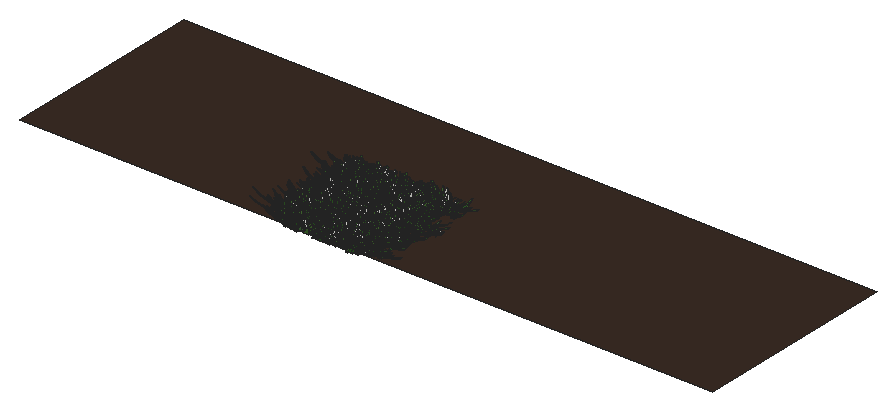
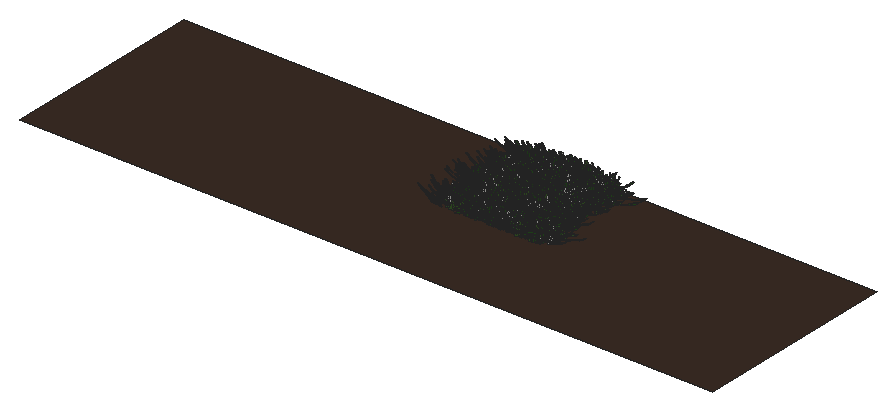
# SketchUp Ruby script. Lengths in inches.
U = 1.inch
M = Sketchup.active_model
def pt(a) = Geom::Point3d.new(a.map { |v| v * U })
def face(e, loops, mat)
  f = e.add_face(loops[0].map { |a| pt(a) })
  loops[1..].each { |l| e.add_face(l.map { |a| pt(a) }).erase! }
  f.material = f.back_material = mat if mat
  f
end
# faces: each face lists its corners as indices into pts; further lists are holes
def faces(e, pts, list, mat = nil) = list.each { |f| face(e, (f[0].is_a?(Array) ? f : [f]).map { |l| l.map { |i| pts[i] } }, mat) }
# xy, xz, yz: faces in a plane at the given z, y or x. An outline is a flat list of corners, or four numbers for a rectangle; further outlines are holes
def ring(l) = l.size == 4 ? [[l[0], l[1]], [l[2], l[1]], [l[2], l[3]], [l[0], l[3]]] : l.each_slice(2).to_a
def flat(e, list, mat, &to3) = list.each { |f| face(e, (f[0].is_a?(Array) ? f : [f]).map { |l| ring(l).map { |u, v| to3.(u, v) } }, mat) }
def xy(e, z, list, mat = nil) = flat(e, list, mat) { |x, y| [x, y, z] }
def xz(e, y, list, mat = nil) = flat(e, list, mat) { |x, z| [x, y, z] }
def yz(e, x, list, mat = nil) = flat(e, list, mat) { |y, z| [x, y, z] }
def lines(e, pts, list) = list.each { |a, b| e.add_line(pt(pts[a]), pt(pts[b])) }
# prism: a flat outline (further loops are holes) pulled along v
def prism(e, loops, v, mat = nil)
  f = face(e, loops, mat); d = Geom::Vector3d.new(v.map { |x| x * U })
  f.pushpull(f.normal.samedirection?(d) ? d.length : -d.length)
end
def box(e, o, s, mat = nil) = prism(e, [[o, [o[0] + s[0], o[1], o[2]], [o[0] + s[0], o[1] + s[1], o[2]], [o[0], o[1] + s[1], o[2]]]], [0, 0, s[2]], mat)
def at(x, y, z, deg = 0) = Geom::Transformation.translation(pt([x, y, z])) * Geom::Transformation.rotation(ORIGIN, Z_AXIS, deg.degrees)
def axes(o, x, y, z) = Geom::Transformation.new([*x, 0, *y, 0, *z, 0, *pt(o).to_a, 1])
def part(name) = M.definitions.add(name)
# library, detail: a bought-in or finely detailed component or shape, given as its bounding box
def library(name, o, s) = part(name).tap { |d| box(d.entities, o, s) }
def detail(e, o, s) = box(e.add_group.entities, o, s)
def put(e, d, t, mat = nil) = e.add_instance(d, t).tap { |i| i.material = mat if mat }
def group(e, t, mat = nil) = e.add_group.tap { |g| g.transformation = t; g.material = mat if mat }.entities
root = M.entities
M.materials.add("Material10").color = [48, 100, 38]
M.materials.add("Material3").color = [68, 110, 58]
M.materials.add("Material4").color = [48, 90, 38]
M.materials.add("Material5").color = [68, 110, 48]
M.materials.add("Material6").color = [48, 90, 48]
M.materials.add("Material7").color = [58, 110, 58]
M.materials.add("Material8").color = [58, 90, 38]
M.materials.add("Material9").color = [68, 100, 58]
M.materials.add("top-soil").color = [58, 44, 36]
c1 = part("grass00")
p = [[-0.6875,0.15,0],[-0.56,0.08,5.52],[-0.04,0.03,2.76],[0.48,-0.02,0],[0.35,-0.02,5.52],[-0.1,-0.14,5.52],
  [-0.12,0.65,8.37],[-0.42,0.65,8.37]]
faces(c1.entities,p,[[0,1,2,3],[3,2,4],[1,5,2],[5,4,2],[1,6,5],[4,5,6],[7,6,1]])
c2 = part("Group16\#1")
put(c2.entities,c1,axes([1.44,-0.61,-0.01],[0.05352,0.12609,0],[-0.10704,0.04543,0.07239],[0.06664,-0.02828,0.11628]),"Material6")
put(c2.entities,c1,axes([0.76,-0.15,-0.01],[0.04676,0.24062,0],[-0.23162,0.04501,0.06642],[0.0652,-0.01267,0.23595]),"Material3")
put(c2.entities,c1,axes([0.79,0.01,-0.01],[-0.00606,0.34651,0],[-0.34381,-0.00602,0.0432],[0.04319,0.00076,0.34386]))
put(c2.entities,c1,axes([1,0.23,-0.01],[-0.07192,0.31144,0],[-0.28722,-0.06632,0.1236],[0.12043,0.02781,0.29478]),"Material5")
put(c2.entities,c1,axes([1.66,0.77,-0.01],[-0.13828,0.29651,0],[-0.21551,-0.1005,0.22471],[0.20365,0.09498,0.23779]),"Material10")
put(c2.entities,c1,axes([0.6875,0.52,-0.01],[-0.18126,0.24051,0],[-0.22746,-0.17142,0.09788],[0.07817,0.05891,0.28481]),"Material5")
put(c2.entities,c1,axes([0.68,0.78,-0.01],[-0.215,0.18688,0],[-0.12385,-0.14248,0.21334],[0.13995,0.16101,0.18878]),"Material3")
put(c2.entities,c1,axes([0.56,1,-0.01],[-0.13756,0.07624,0],[-0.06159,-0.11112,0.0927],[0.04494,0.08108,0.12705]),"Material5")
put(c2.entities,c1,axes([0.2,0.64,-0.01],[-0.23729,0.07254,0],[-0.05711,-0.18681,0.153],[0.04473,0.14632,0.19535]),"Material10")
put(c2.entities,c1,axes([0.0625,0.72,-0.01],[-0.28874,0.02525,0],[-0.02179,-0.24916,0.14647],[0.01276,0.14591,0.25012]),"Material3")
put(c2.entities,c1,axes([-0.08,0.62,-0.01],[-0.34089,-0.04187,0],[0.03255,-0.26504,0.216],[-0.02633,0.21439,0.26703]),"Material10")
put(c2.entities,c1,axes([-0.34,0.98,-0.01],[-0.14314,-0.0493,0],[0.04397,-0.12769,0.06843],[-0.02228,0.0647,0.13505]),"Material10")
put(c2.entities,c1,axes([-0.87,1.45,-0.01],[-0.23488,-0.14114,0],[0.13761,-0.22901,0.06087],[-0.03135,0.05217,0.26717]))
put(c2.entities,c1,axes([-0.72,0.77,-0.01],[-0.14208,-0.13251,0],[0.07209,-0.0773,0.16301],[-0.11118,0.11922,0.1057]),"Material10")
put(c2.entities,c1,axes([-0.62,0.43,-0.01],[-0.14845,-0.21203,0],[0.18654,-0.13061,0.12304],[-0.10079,0.07057,0.22772]),"Material3")
put(c2.entities,c1,axes([-0.68,0.29,-0.01],[-0.13639,-0.32136,0],[0.31723,-0.13464,0.05579],[-0.05136,0.0218,0.34462]),"Material4")
put(c2.entities,c1,axes([-0.64,0.125,-0.01],[-0.0458,-0.23569,0],[0.22124,-0.043,0.08276],[-0.08124,0.01579,0.22538]),"Material7")
put(c2.entities,c1,axes([-1.6,-0.03,-0.01],[0.00576,-0.32897,0],[0.27526,0.00482,0.18018],[-0.18015,-0.00315,0.2753]),"Material5")
put(c2.entities,c1,axes([-1.36,-0.31,-0.01],[0.05718,-0.24765,0],[0.18172,0.04196,0.17267],[-0.16825,-0.03885,0.1865]),"Material10")
put(c2.entities,c1,axes([-1.54,-0.72,-0.01],[0.06537,-0.14017,0],[0.13555,0.06321,0.03939],[-0.0357,-0.01665,0.14956]))
put(c2.entities,c1,axes([-1.19,-0.9,-0.01],[0.09597,-0.12735,0],[0.11214,0.08451,0.07557],[-0.06035,-0.04548,0.14042]),"Material9")
put(c2.entities,c1,axes([-0.47,-0.54,-0.01],[0.11588,-0.10072,0],[0.0618,0.0711,0.12124],[-0.07953,-0.0915,0.0942]))
put(c2.entities,c1,axes([-0.47,-0.84,-0.01],[0.11927,-0.0661,0],[0.06603,0.11913,0.00646],[-0.00313,-0.00565,0.13621]),"Material5")
put(c2.entities,c1,axes([-0.38,-1.24,-0.01],[0.28037,-0.08571,0],[0.0618,0.20215,0.20315],[-0.05939,-0.19428,0.21139]),"Material9")
put(c2.entities,c1,axes([-0.06,-0.66,-0.01],[0.22719,-0.01987,0],[0.01247,0.14255,0.17758],[-0.01547,-0.17691,0.1431]),"Material8")
put(c2.entities,c1,axes([0.11,-0.89,-0.01],[0.14882,0.01828,0],[-0.01058,0.08611,0.12229],[0.01491,-0.12138,0.08676]),"Material6")
put(c2.entities,c1,axes([0.25,-0.72,-0.01],[0.20481,0.07053,0],[-0.06206,0.18022,0.10291],[0.03351,-0.0973,0.1906]),"Material6")
put(c2.entities,c1,axes([0.85,-1.42,-0.01],[0.16481,0.09904,0],[-0.09472,0.15762,0.05616],[0.02893,-0.04814,0.18389]),"Material5")
put(c2.entities,c1,axes([1.01,-1.09,-0.01],[0.21858,0.20385,0],[-0.17495,0.1876,0.15339],[0.10462,-0.11218,0.25652]),"Material10")
put(c2.entities,c1,axes([1.01,-0.71,-0.01],[0.08733,0.12473,0],[-0.06445,0.04512,0.13037],[0.1068,-0.07477,0.07867]),"Material6")
c3 = part("Group15\#1")
put(c3.entities,c2,at(0,0,0))
c4 = part("3darcstudiotree_grass00\#1")
put(c4.entities,c3,at(0,0,0))
xy(root,7.6,[[26,3.94,292.14,82.68]],"top-soil")
put(root,c4,axes([127.27,11.34,7.6],[-4.63896,0.21302,0],[-0.93332,-1.27031,-0.05609],[-0.06093,-0.08294,1.94158]))
put(root,c4,axes([127.55,18.1,7.6],[-4.20413,-0.53147,0],[1.63067,-0.8062,-0.0255],[0.09899,-0.04894,1.94297]))
put(root,c4,axes([127.2,43.18,7.6],[-3.5275,0.23131,0],[-1.26087,-1.2018,-0.03948],[-0.051,-0.04861,1.58152]))
put(root,c4,axes([127.18,37.69,7.6],[-3.90893,0.68034,0],[-2.78299,-0.99937,-0.02528],[-0.08388,-0.03012,1.76765]))
put(root,c4,axes([126.91,8.79,7.6],[0.1527,1.05059,0],[-3.86386,0.0351,-0.04285],[-0.32383,0.00294,1.82733]))
put(root,c4,axes([127.11,36.11,7.6],[3.71157,-0.27079,0],[1.39023,1.19096,-0.04654],[0.05647,0.04838,1.34343]))
put(root,c4,axes([126.82,41.7,7.6],[3.97715,0.44667,0],[-1.63668,0.9108,-0.04301],[-0.1186,0.066,1.6797]))
put(root,c4,axes([127.44,18.69,7.6],[3.86502,-0.35215,0],[1.63703,1.12296,-0.06136],[0.12705,0.08716,1.80687]))
put(root,c4,axes([128.97,10.05,7.6],[-0.56967,-1.02254,0],[3.9547,-0.1377,-0.01078],[0.07697,-0.00268,1.79898]))
put(root,c4,axes([129.37,26.41,7.6],[-1.46525,-0.90866,0],[3.94836,-0.39793,-0.00075],[0.00398,-0.0004,1.52674]))
put(root,c4,axes([127.8,13.4,7.6],[4.11417,0.05124,0],[-0.24086,1.20875,-0.00527],[-0.00138,0.00693,1.59512]))
put(root,c4,axes([130.11,40.14,7.6],[-2.16831,-1.16182,0],[4.23849,-0.49439,-0.01753],[0.08143,-0.0095,1.49864]))
put(root,c4,axes([128.8,31.7,7.6],[3.83036,-0.81769,0],[2.5645,0.75081,-0.01134],[0.04499,0.01317,1.5074]))
put(root,c4,axes([129.61,7.45,7.6],[-4.70771,0.35936,0],[-1.47237,-1.20555,-0.03433],[-0.04305,-0.03525,1.35329]))
put(root,c4,axes([129.38,27.65,7.6],[-3.29867,0.81125,0],[-2.71253,-0.68934,-0.0233],[-0.12397,-0.0315,1.83382]))
put(root,c4,axes([129.1,29.73,7.6],[-0.78138,1.08578,0],[-4.54266,-0.20432,-0.02584],[-0.11477,-0.00516,1.30174]))
put(root,c4,axes([130.37,33.88,7.6],[2.17808,-0.78505,0],[4.26827,0.74013,-0.02169],[0.08641,0.01498,1.57389]))
put(root,c4,axes([129.44,14.47,7.6],[-0.70651,0.89155,0],[-4.48869,-0.22232,-0.03573],[-0.20534,-0.01017,1.67549]))
put(root,c4,axes([130.97,5.17,7.6],[-3.74457,-0.22418,0],[0.88563,-0.92456,-0.00326],[0.00619,-0.00646,1.93944]))
put(root,c4,axes([129.33,16.31,7.6],[3.07381,0.68375,0],[-2.58138,0.72529,-0.00943],[-0.03598,0.01011,1.39243]))
put(root,c4,axes([130.14,21.73,7.6],[-0.98652,1.16576,0],[-4.8711,-0.25764,-0.05558],[-0.27807,-0.01471,1.59125]))
put(root,c4,axes([130.92,38.5,7.6],[1.84217,-1.02173,0],[3.32278,0.37443,-0.02223],[0.14494,0.01633,1.62899]))
put(root,c4,axes([131.01,32.25,7.6],[3.84212,-0.38705,0],[1.37613,0.85378,-0.02314],[0.05053,0.03135,1.34449]))
put(root,c4,axes([130.4375,23.45,7.6],[1.9287,1.10406,0],[-3.72338,0.40653,-0.01938],[-0.11115,0.01214,1.58937]))
put(root,c4,axes([132.83,17.88,7.6],[-1.7561,-0.89869,0],[3.62331,-0.44251,-0.0349],[0.22933,-0.02801,1.84302]))
put(root,c4,axes([133.47,27.125,7.6],[-4.2283,-0.0064,0],[0.03055,-1.26138,-0.0591],[0.00173,-0.07136,1.52309]))
put(root,c4,axes([133.69,24.17,7.6],[-4.7095,-0.098,0],[0.36806,-1.10545,-0.036],[0.02101,-0.06311,1.9513]))
put(root,c4,axes([133.45,35.24,7.6],[1.82992,-1.20621,0],[3.40004,0.32238,-0.00605],[0.04862,0.00461,1.95327]))
put(root,c4,axes([133.55,43.5,7.6],[1.45443,-0.84507,0],[4.00274,0.43056,-0.02985],[0.15547,0.01672,1.54439]))
put(root,c4,axes([133.23,32.14,7.6],[0.91767,-0.96683,0],[3.51247,0.20837,-0.04624],[0.38905,0.02308,1.95114]))
put(root,c4,axes([133.22,38.91,7.6],[-2.22547,0.97496,0],[-3.23871,-0.46204,-0.04437],[-0.2422,-0.03455,1.46464]))
put(root,c4,axes([132.83,9.93,7.6],[-1.07117,1.0548,0],[-4.16401,-0.26429,-0.01715],[-0.09038,-0.00574,1.46021]))
put(root,c4,axes([134.55,27.97,7.6],[-0.7412,-1.17343,0],[4.56586,-0.18025,-0.01303],[0.08774,-0.00346,1.96953]))
put(root,c4,axes([134.2,4.24,7.6],[1.34034,-1.07316,0],[4.75764,0.37138,-0.04262],[0.23721,0.01852,1.81655]))
put(root,c4,axes([134.86,20.11,7.6],[-4.70029,0.25343,0],[-0.93391,-1.08255,-0.00845],[-0.00874,-0.01013,1.35873]))
put(root,c4,axes([134.27,12.98,7.6],[-2.69017,1.10468,0],[-3.43594,-0.52296,-0.03488],[-0.16243,-0.02472,1.37068]))
put(root,c4,axes([133.78,16.36,7.6],[3.70476,-0.12271,0],[0.5167,0.975,-0.04905],[0.03883,0.07327,1.48186]))
put(root,c4,axes([134.5,22.14,7.6],[-3.18848,0.90294,0],[-3.14265,-0.69359,-0.01581],[-0.06022,-0.01329,1.33135]))
put(root,c4,axes([134.46,7.4,7.6],[3.51285,-0.33152,0],[1.41112,0.93454,-0.04981],[0.11878,0.07867,1.68613]))
put(root,c4,axes([135.81,7.89,7.6],[-0.91328,-1.0252,0],[3.54973,-0.19764,-0.00779],[0.04648,-0.00259,1.38852]))
put(root,c4,axes([135.84,25.51,7.6],[-2.2581,-1.00308,0],[3.75758,-0.52868,-0.05229],[0.27859,-0.0392,1.64764]))
put(root,c4,axes([135.94,14.56,7.6],[0.44969,-0.9198,0],[4.71868,0.14419,-0.02785],[0.1393,0.00426,1.49696]))
put(root,c4,axes([134.95,19.14,7.6],[-2.40206,1.15116,0],[-4.41351,-0.57559,-0.04188],[-0.22518,-0.02937,1.88687]))
put(root,c4,axes([134.27,34.35,7.6],[3.15973,0.64464,0],[-2.80076,0.858,-0.03119],[-0.13565,0.04156,1.90467]))
put(root,c4,axes([135.51,41.9375,7.6],[-2.00451,1.10371,0],[-3.34752,-0.37998,-0.0444],[-0.28643,-0.03251,1.62807]))
put(root,c4,axes([135.89,29.28,7.6],[-2.48346,0.94681,0],[-4.13972,-0.67865,-0.05216],[-0.1846,-0.03026,1.30947]))
put(root,c4,axes([135.89,30.77,7.6],[-2.01885,1.11907,0],[-4.67604,-0.52724,-0.03185],[-0.16487,-0.01859,1.82087]))
put(root,c4,axes([135.99,11.52,7.6],[2.27461,0.70298,0],[-2.88603,0.58364,-0.02717],[-0.1658,0.03353,1.82093]))
put(root,c4,axes([136.1,5.39,7.6],[3.78924,0.26456,0],[-0.97261,0.87066,-0.03829],[-0.06398,0.05727,1.40372]))
put(root,c4,axes([136.66,37.57,7.6],[4.35332,-0.20638,0],[0.96031,1.26603,-0.05959],[0.0538,0.07093,1.56123]))
put(root,c4,axes([136.8,39.91,7.6],[0.89231,1.23104,0],[-4.86402,0.22035,-0.02342],[-0.12734,0.00577,1.70718]))
put(root,c4,axes([139.1,5.15,7.6],[-3.95423,-0.27375,0],[1.31501,-1.1872,-0.02644],[0.04369,-0.03944,1.9068]))
put(root,c4,axes([139.88,32.84,7.6],[-4.2551,-0.55246,0],[2.21747,-1.06745,-0.03725],[0.08878,-0.04274,1.55507]))
put(root,c4,axes([139.01,41.67,7.6],[-2.9637,1.00971,0],[-3.98182,-0.73047,-0.06171],[-0.27775,-0.05095,1.72322]))
put(root,c4,axes([138.73,36.84,7.6],[1.86969,0.78057,0],[-3.16238,0.47343,-0.04808],[-0.33365,0.04995,1.86326]))
put(root,c4,axes([138.69,24.79,7.6],[4.806,-0.14737,0],[0.47152,0.96109,-0.03723],[0.02452,0.04998,1.30959]))
put(root,c4,axes([140.17,38.59,7.6],[0.365,-1.172,0],[4.21149,0.08198,-0.01871],[0.12678,0.00247,1.79426]))
put(root,c4,axes([140.74,26.9,7.6],[-2.38517,-0.85712,0],[3.89197,-0.67691,-0.03629],[0.14533,-0.02528,1.44541]))
put(root,c4,axes([140.84,23.5,7.6],[-2.55212,-0.67388,0],[3.75826,-0.88958,-0.06171],[0.2261,-0.05352,1.63202]))
put(root,c4,axes([141.06,8.08,7.6],[0.94935,-1.13668,0],[4.79838,0.25048,-0.01659],[0.08229,0.0043,1.55232]))
put(root,c4,axes([141.66,34.77,7.6],[-4.47557,-0.42377,0],[1.78381,-1.17745,-0.00084],[0.00126,-0.00083,1.34285]))
put(root,c4,axes([140.8,31.3,7.6],[-2.98855,0.54778,0],[-2.22427,-0.75844,-0.03589],[-0.17423,-0.05941,1.93035]))
put(root,c4,axes([140.2,30.07,7.6],[3.78365,-0.18577,0],[0.80923,1.03012,-0.00241],[0.00316,0.00403,1.79003]))
put(root,c4,axes([140.74,28.52,7.6],[-1.65227,1.03376,0],[-3.9595,-0.39553,-0.0529],[-0.2919,-0.02916,1.58349]))
put(root,c4,axes([140.19,15.65,7.6],[1.52496,0.98405,0],[-3.48981,0.338,-0.02409],[-0.15435,0.01495,1.60735]))
put(root,c4,axes([140.0625,7.08,7.6],[5.01381,0.29286,0],[-0.86637,0.92702,-0.04207],[-0.05348,0.05723,1.32997]))
put(root,c4,axes([141.42,12.63,7.6],[-3.05375,0.95057,0],[-3.1621,-0.6349,-0.04358],[-0.22353,-0.04488,1.66757]))
put(root,c4,axes([140.66,21.92,7.6],[3.93232,0.3892,0],[-1.53002,0.96616,-0.03237],[-0.07493,0.04731,1.63378]))
put(root,c4,axes([141.875,43.1,7.6],[-3.88658,0.80784,0],[-2.79245,-0.83967,-0.00935],[-0.03544,-0.01066,1.61847]))
put(root,c4,axes([141.68,20.12,7.6],[3.7138,-0.79833,0],[2.34942,0.68309,-0.0226],[0.10849,0.03154,1.65792]))
put(root,c4,axes([142.91,36.16,7.6],[-4.61826,-0.0324,0],[0.10564,-0.94117,-0.03959],[0.00926,-0.08249,1.96257]))
put(root,c4,axes([141.23,19.13,7.6],[4.49063,0.58178,0],[-2.32504,1.12165,-0.0509],[-0.11953,0.05767,1.61215]))
put(root,c4,axes([141.99,17.91,7.6],[4.04347,-0.18678,0],[0.90955,1.23062,-0.01263],[0.0127,0.01719,1.73191]))
put(root,c4,axes([142.74,11.63,7.6],[3.03325,-1.05553,0],[3.12611,0.56147,-0.0087],[0.04718,0.00847,1.60603]))
put(root,c4,axes([142.99,14.52,7.6],[3.36364,-0.39705,0],[1.75914,0.93141,-0.03456],[0.09555,0.05059,1.66747]))
put(root,c4,axes([143.09,39.81,7.6],[-0.83011,0.88053,0],[-3.59902,-0.21206,-0.04738],[-0.28817,-0.01698,1.4441]))
put(root,c4,axes([142.34,10.4375,7.6],[2.92685,0.95557,0],[-3.59966,0.68909,-0.02004],[-0.07664,0.01467,1.3651]))
put(root,c4,axes([144.82,43.36,7.6],[-3.93046,0.12235,0],[-0.4536,-0.91071,-0.03309],[-0.02864,-0.0575,1.60704]))
put(root,c4,axes([145.28,29.79,7.6],[-3.8765,-0.37875,0],[1.47892,-0.94605,-0.02269],[0.05344,-0.03418,1.64292]))
put(root,c4,axes([145.06,11.28,7.6],[-4.50586,0.35674,0],[-1.23927,-0.9783,-0.01419],[-0.02922,-0.02307,1.75006]))
put(root,c4,axes([144.87,4.05,7.6],[2.37725,-0.90712,0],[3.87375,0.63448,-0.04807],[0.23586,0.03863,1.69791]))
put(root,c4,axes([145.04,20.64,7.6],[2.75939,-0.81589,0],[3.35102,0.70833,-0.03628],[0.15055,0.03182,1.49031]))
put(root,c4,axes([145.93,35.41,7.6],[-1.86432,-1.00241,0],[3.34424,-0.38873,-0.04244],[0.31797,-0.03696,1.90455]))
put(root,c4,axes([145.94,5.34,7.6],[1.78946,-1.14425,0],[3.5583,0.3478,-0.00888],[0.06487,0.00634,1.87213]))
put(root,c4,axes([144.92,6.41,7.6],[-1.11444,1.02351,0],[-4.99646,-0.34002,-0.0223],[-0.10571,-0.00719,1.58974]))
put(root,c4,axes([146.7,40.54,7.6],[-1.04914,-1.06304,0],[3.77307,-0.23273,-0.01268],[0.08139,-0.00502,1.60602]))
put(root,c4,axes([147.2,21.73,7.6],[-2.07823,-1.0748,0],[4.05386,-0.48991,-0.04214],[0.21023,-0.02541,1.55921]))
put(root,c4,axes([146.41,36.81,7.6],[-3.28261,0.64166,0],[-2.52163,-0.80626,-0.02144],[-0.10036,-0.03209,1.94421]))
put(root,c4,axes([145.77,26.5,7.6],[-0.6945,0.99441,0],[-4.06846,-0.17759,-0.03794],[-0.20649,-0.00901,1.42617]))
put(root,c4,axes([146.39,9.59,7.6],[-2.06095,0.96891,0],[-3.40314,-0.45242,-0.04799],[-0.3505,-0.0466,1.99284]))
put(root,c4,axes([147.52,16.39,7.6],[-2.17627,-1.09913,0],[3.44474,-0.42628,-0.01272],[0.06522,-0.00807,1.37453]))
put(root,c4,axes([147.27,41.53,7.6],[0.22128,-1.19645,0],[4.67967,0.05409,-0.04434],[0.23423,0.00271,1.54852]))
put(root,c4,axes([148.22,17.7,7.6],[-3.09718,-0.64135,0],[2.64207,-0.79743,-0.01497],[0.06729,-0.02031,1.82381]))
put(root,c4,axes([146.64,7.95,7.6],[-1.82154,1.01586,0],[-4.52061,-0.50662,-0.00369],[-0.01716,-0.00192,1.57624]))
put(root,c4,axes([147.45,14.75,7.6],[-3.65354,0.89474,0],[-2.56614,-0.6549,-0.00183],[-0.00785,-0.002,1.40539]))
put(root,c4,axes([147.26,31.32,7.6],[-2.50195,1.12274,0],[-4.19712,-0.58456,-0.0557],[-0.2512,-0.03499,1.55009]))
put(root,c4,axes([148.65,33.93,7.6],[-3.5144,-0.95148,0],[3.77994,-0.8726,-0.04946],[0.16772,-0.03872,1.48426]))
put(root,c4,axes([148.45,24.66,7.6],[-4.39725,-0.1693,0],[0.59529,-0.96636,-0.03709],[0.03896,-0.06324,1.68681]))
put(root,c4,axes([148.07,23.46,7.6],[-3.41733,0.39454,0],[-1.99566,-1.08035,-0.05064],[-0.10494,-0.05681,1.47033]))
put(root,c4,axes([148.89,13.12,7.6],[0.92698,-1.20285,0],[4.36209,0.2101,-0.00212],[0.01245,0.0006,1.6588]))
put(root,c4,axes([148.24,38.7,7.6],[3.47512,-0.34723,0],[1.8254,1.14182,-0.02256],[0.04248,0.02657,1.55958]))
put(root,c4,axes([148.79,32.17,7.6],[2.15551,-0.74125,0],[3.38784,0.61573,-0.02782],[0.16259,0.02955,1.89124]))
put(root,c4,axes([148.2,19.44,7.6],[2.61248,0.6584,0],[-3.28353,0.8143,-0.03885],[-0.15165,0.03761,1.58937]))
put(root,c4,axes([148.8,28.62,7.6],[3.40608,0.31789,0],[-1.62863,1.09064,-0.03179],[-0.06759,0.04526,1.76952]))
put(root,c4,axes([150.89,25.37,7.6],[-1.7547,-0.95302,0],[3.61048,-0.41547,-0.04546],[0.29745,-0.03423,1.78943]))
put(root,c4,axes([151.28,26.83,7.6],[1.053,-0.96727,0],[3.62694,0.24678,-0.01758],[0.12396,0.00843,1.71636]))
put(root,c4,axes([151.69,11.54,7.6],[-3.98559,-0.40727,0],[1.42948,-0.87432,-0.04864],[0.11159,-0.06825,1.4319]))
put(root,c4,axes([151.83,32.16,7.6],[-1.88311,-0.95255,0],[4.51474,-0.55783,-0.04891],[0.26234,-0.03241,1.88309]))
put(root,c4,axes([152.09,41.46,7.6],[-4.25078,-0.391,0],[1.69928,-1.15461,-0.01333],[0.0258,-0.01753,1.7245]))
put(root,c4,axes([151.35,43.3,7.6],[-3.78924,0.73867,0],[-2.26636,-0.72662,-0.02241],[-0.08836,-0.02833,1.47722]))
put(root,c4,axes([151.625,9.9,7.6],[-0.58963,-1.12221,0],[3.81516,-0.12529,-0.04534],[0.30342,-0.00996,1.62314]))
put(root,c4,axes([152.04,19.02,7.6],[0.02643,-0.92207,0],[3.81186,0.00683,-0.01704],[0.12849,0.00023,1.79616]))
put(root,c4,axes([150.75,39.88,7.6],[-1.16899,0.9922,0],[-4.24579,-0.31264,-0.01201],[-0.06083,-0.00448,1.46096]))
put(root,c4,axes([152.48,23.07,7.6],[-1.37406,-1.03466,0],[4.06189,-0.33714,-0.03393],[0.15904,-0.0132,1.3212]))
put(root,c4,axes([151.27,4.06,7.6],[4.45768,-0.32922,0],[1.38468,1.17179,-0.05518],[0.09073,0.07678,1.77288]))
put(root,c4,axes([153,7,7.6],[1.09423,-1.18623,0],[4.14621,0.23904,-0.00305],[0.01978,0.00114,1.76865]))
put(root,c4,axes([152.11,20.95,7.6],[-2.60907,0.74079,0],[-3.52374,-0.77567,-0.02335],[-0.09985,-0.02198,1.67208]))
put(root,c4,axes([151.37,34.32,7.6],[0.14823,0.94449,0],[-4.53661,0.0445,-0.00595],[-0.04152,0.00041,1.98232]))
put(root,c4,axes([152.59,35.5625,7.6],[-3.76988,0.83286,0],[-3.11368,-0.88087,-0.04086],[-0.13444,-0.03803,1.46035]))
put(root,c4,axes([152.85,21.7,7.6],[2.7445,-0.91806,0],[3.21973,0.60158,-0.03861],[0.21673,0.04049,1.76068]))
put(root,c4,axes([153.68,7.92,7.6],[0.91501,-1.15723,0],[4.8883,0.24157,-0.04547],[0.24719,0.01222,1.72572]))
put(root,c4,axes([153.45,39.02,7.6],[-4.13262,0.75948,0],[-2.24844,-0.76466,-0.00523],[-0.01922,-0.00654,1.47184]))
put(root,c4,axes([153.48,28.48,7.6],[-3.86969,0.48099,0],[-1.95079,-0.98092,-0.01143],[-0.02514,-0.01264,1.35283]))
put(root,c4,axes([152.52,14.34,7.6],[3.86312,0.38228,0],[-1.39067,0.87833,-0.04887],[-0.14094,0.08902,1.85053]))
put(root,c4,axes([154.58,16.12,7.6],[-4.70177,-0.53336,0],[2.03054,-1.11874,-0.00153],[0.00375,-0.00206,1.82565]))
put(root,c4,axes([154.29,5.44,7.6],[-4.46822,-0.10581,0],[0.37585,-0.99198,-0.02721],[0.01358,-0.03584,1.31849]))
put(root,c4,axes([153.13,30.65,7.6],[1.40657,1.03003,0],[-3.82031,0.32605,-0.04031],[-0.26799,0.02287,1.77227]))
put(root,c4,axes([154.25,37.61,7.6],[-3.92611,0.32664,0],[-1.54996,-1.16439,-0.02244],[-0.03763,-0.02827,1.62972]))
put(root,c4,axes([154.62,18.04,7.6],[0.29188,-1.2036,0],[4.4228,0.06704,-0.02606],[0.15802,0.0024,1.68211]))
put(root,c4,axes([154.32,13.34,7.6],[-2.65492,0.94025,0],[-3.53882,-0.62452,-0.04566],[-0.22738,-0.04013,1.65042]))
put(root,c4,axes([155.15,29.9375,7.6],[4.17906,-0.20511,0],[0.89097,1.13456,-0.02697],[0.02876,0.03662,1.59996]))
put(root,c4,axes([157.64,19.14,7.6],[-4.41351,-0.36972,0],[1.24316,-0.9275,-0.02118],[0.04591,-0.03425,1.66873]))
put(root,c4,axes([158.16,15.46,7.6],[0.53348,-0.96081,0],[3.98331,0.13823,-0.0013],[0.00952,0.00033,1.85519]))
put(root,c4,axes([157.46,41.31,7.6],[-1.33514,1.21073,0],[-3.80153,-0.26201,-0.03305],[-0.17466,-0.01204,1.35106]))
put(root,c4,axes([158.09,28.41,7.6],[-2.22446,1.02155,0],[-4.2399,-0.57703,-0.05406],[-0.24223,-0.03297,1.53936]))
put(root,c4,axes([157.29,13.06,7.6],[1.18915,1.16091,0],[-4.66954,0.29894,-0.00469],[-0.02419,0.00155,1.60422]))
put(root,c4,axes([158.92,26.89,7.6],[-3.71937,0.41864,0],[-1.99025,-1.10514,-0.05685],[-0.1451,-0.08057,1.88376]))
put(root,c4,axes([158.2,6.48,7.6],[-0.88189,0.99912,0],[-4.57623,-0.25246,-0.05256],[-0.22927,-0.01265,1.30827]))
put(root,c4,axes([159.09,39.18,7.6],[1.87855,-0.80281,0],[3.39229,0.49612,-0.02347],[0.15921,0.02328,1.9305]))
put(root,c4,axes([159.83,25.47,7.6],[-0.60906,-0.96226,0],[5.07736,-0.20086,-0.05346],[0.24254,-0.00959,1.47567]))
put(root,c4,axes([158.25,43.37,7.6],[-0.43739,1.1748,0],[-4.7805,-0.11124,-0.02425],[-0.1421,-0.00331,1.76617]))
